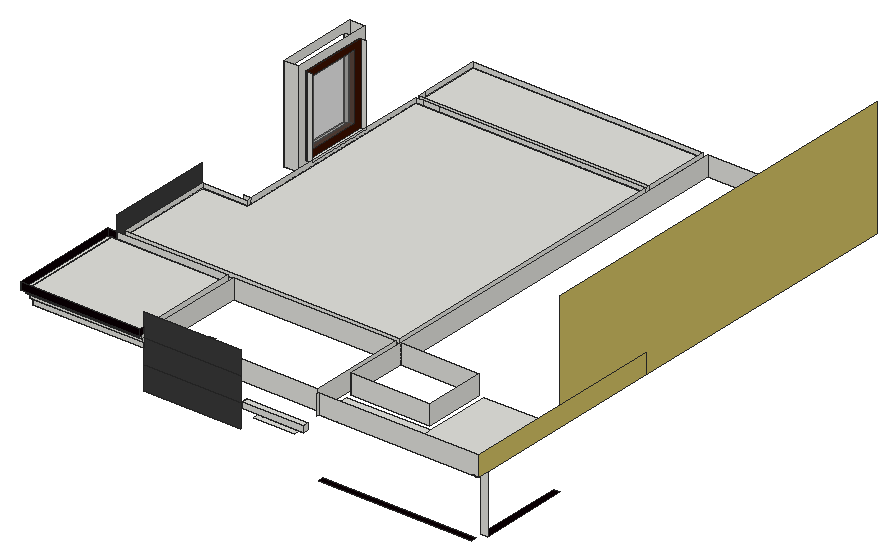
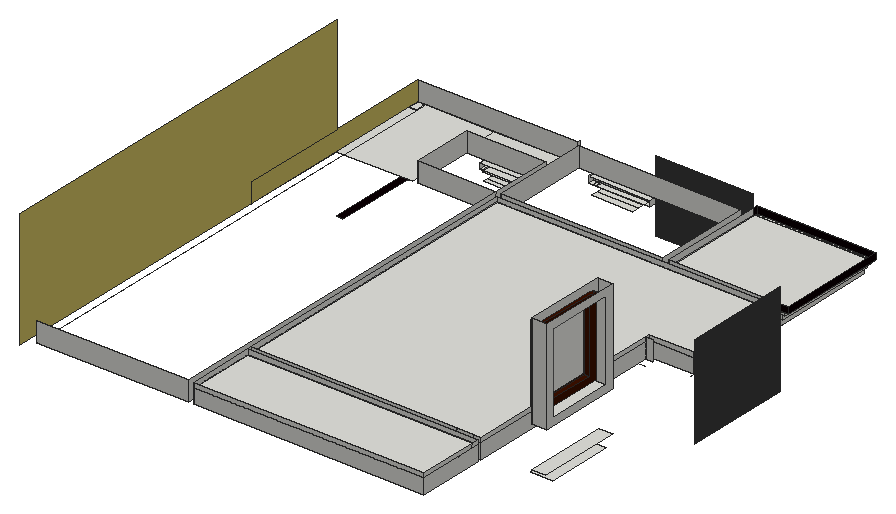
# SketchUp Ruby script. Lengths in inches.
U = 1.inch
M = Sketchup.active_model
def pt(a) = Geom::Point3d.new(a.map { |v| v * U })
def face(e, loops, mat)
  f = e.add_face(loops[0].map { |a| pt(a) })
  loops[1..].each { |l| e.add_face(l.map { |a| pt(a) }).erase! }
  f.material = f.back_material = mat if mat
  f
end
# faces: each face lists its corners as indices into pts; further lists are holes
def faces(e, pts, list, mat = nil) = list.each { |f| face(e, (f[0].is_a?(Array) ? f : [f]).map { |l| l.map { |i| pts[i] } }, mat) }
# xy, xz, yz: faces in a plane at the given z, y or x. An outline is a flat list of corners, or four numbers for a rectangle; further outlines are holes
def ring(l) = l.size == 4 ? [[l[0], l[1]], [l[2], l[1]], [l[2], l[3]], [l[0], l[3]]] : l.each_slice(2).to_a
def flat(e, list, mat, &to3) = list.each { |f| face(e, (f[0].is_a?(Array) ? f : [f]).map { |l| ring(l).map { |u, v| to3.(u, v) } }, mat) }
def xy(e, z, list, mat = nil) = flat(e, list, mat) { |x, y| [x, y, z] }
def xz(e, y, list, mat = nil) = flat(e, list, mat) { |x, z| [x, y, z] }
def yz(e, x, list, mat = nil) = flat(e, list, mat) { |y, z| [x, y, z] }
def lines(e, pts, list) = list.each { |a, b| e.add_line(pt(pts[a]), pt(pts[b])) }
# prism: a flat outline (further loops are holes) pulled along v
def prism(e, loops, v, mat = nil)
  f = face(e, loops, mat); d = Geom::Vector3d.new(v.map { |x| x * U })
  f.pushpull(f.normal.samedirection?(d) ? d.length : -d.length)
end
def box(e, o, s, mat = nil) = prism(e, [[o, [o[0] + s[0], o[1], o[2]], [o[0] + s[0], o[1] + s[1], o[2]], [o[0], o[1] + s[1], o[2]]]], [0, 0, s[2]], mat)
def at(x, y, z, deg = 0) = Geom::Transformation.translation(pt([x, y, z])) * Geom::Transformation.rotation(ORIGIN, Z_AXIS, deg.degrees)
def axes(o, x, y, z) = Geom::Transformation.new([*x, 0, *y, 0, *z, 0, *pt(o).to_a, 1])
def part(name) = M.definitions.add(name)
# library, detail: a bought-in or finely detailed component or shape, given as its bounding box
def library(name, o, s) = part(name).tap { |d| box(d.entities, o, s) }
def detail(e, o, s) = box(e.add_group.entities, o, s)
def put(e, d, t, mat = nil) = e.add_instance(d, t).tap { |i| i.material = mat if mat }
def group(e, t, mat = nil) = e.add_group.tap { |g| g.transformation = t; g.material = mat if mat }.entities
root = M.entities
M.materials.add("[Color C08]").color = [60, 17, 0]
M.materials.add("[Color D05]").color = [208, 191, 99]
M.materials.add("[Color M07]").color = [58, 58, 58]
M.materials.add("[Metal Seamed]").color = [11, 0, 4]
M.materials.add("[Translucent Glass Gray]").color = [128, 128, 128]
M.materials["[Translucent Glass Gray]"].alpha = 0.5
c1 = part("Group\#2")
xy(c1.entities,0,[[0,0,43.625,4]],"[Color C08]")
xy(c1.entities,4.9,[[4.9,0,38.73,4]],"[Color C08]")
xy(c1.entities,53.48,[[4.9,0,38.73,4]],"[Color C08]")
xy(c1.entities,58.375,[[0,0,43.625,4]],"[Color C08]")
xz(c1.entities,0,[[[0,0,43.625,58.375],[4.9,4.9,38.73,53.48]]],"[Color C08]")
xz(c1.entities,0,[[4.9,4.9,38.73,53.48]],"[Translucent Glass Gray]")
xz(c1.entities,4,[[[0,0,43.625,58.375],[4.9,4.9,38.73,53.48]]],"[Color C08]")
yz(c1.entities,0,[[0,0,4,58.375]],"[Color C08]")
yz(c1.entities,4.9,[[0,4.9,4,53.48]],"[Color C08]")
yz(c1.entities,38.73,[[0,4.9,4,53.48]],"[Color C08]")
yz(c1.entities,43.625,[[0,0,4,58.375]],"[Color C08]")
xy(root,191.0625,[[559.49,92.73,560.01,92.74,560.51,92.9,560.95,93.18,561.31,93.56,561.55,94.02,561.67,94.53,561.65,95.05,561.49,95.55,561.22,95.99,560.83,96.35,560.37,96.59,559.86,96.71,559.34,96.6875,558.84,96.53,558.4,96.26,558.04,95.875,557.8,95.41,557.68,94.9,557.7,94.38,557.86,93.88,558.14,93.44,558.52,93.09,558.98,92.84]])
xy(root,192,[[369.3125,70.41,556.3125,77.3]],"[Metal Seamed]")
xy(root,192.96,[[556.24,84.63,564.3125,195.41]],"[Metal Seamed]")
xy(root,216.84,[[55.1875,419.61,72.6875,501.8],[72.6875,419.61,81.6875,501.8]])
xy(root,227.14,[[55.1875,409.31,72.6875,512.1]])
xy(root,232.4375,[[158,120.11,165.5625,168.11]])
xy(root,239.79,[[297.45,60.85,347.52,67.28],[297.45,67.28,347.52,76.28]])
xy(root,239.92,[[395.02,106.41,445.08,113.66],[395.02,113.66,445.08,119.66]])
xy(root,245.34,[[291.9,60.85,349.28,67.28],[349.28,60.85,353.07,67.28]])
xy(root,245.63,[[283.19,59.85,289.58,67.28],[289.58,59.85,349.28,67.28],[349.28,59.85,359.01,60.85],[353.07,60.85,359.01,67.28]])
xy(root,245.96,[[388.97,106.41,451.12,113.66]])
xy(root,246.98,[[385.19,101.28,391.58,113.66],[451.27,101.28,455.06,113.66]])
xy(root,247.26,[[391.58,101.28,451.27,113.66]])
xy(root,252.66,[[283.19,59.85,359.01,67.28]])
xy(root,254.29,[[385.19,101.28,455.06,113.66]])
xy(root,263.5625,[[24.07,73.08,41.19,92.83]])
xy(root,264,[[21.625,67.66,158,195.41],[556.3,70.41,556.3,70.97,555.3125,70.97,555.3125,195.41,564.5,195.41,564.5,84.63,564.3125,84.63,564.3125,70.41],[369.3125,70.97,471.3125,113.66],[471.3125,70.97,555.3125,195.41],[564.3125,195.41,564.5,326.53]])
xy(root,264.0625,[[556.3,70.41,564.3125,70.97],[556.3,70.97,564.3125,70.97,564.3125,84.63,556.24,84.63,556.3,77.3],[564.3125,70.97,564.5,84.63]])
xy(root,271.375,[[19,65.66,19,195.41,21.625,195.41,21.625,67.66,21.75,67.66,21.75,65.66],[21.75,65.66,158,67.66],[21.625,67.66,158,195.41]])
xy(root,276.0625,[[15.8125,63.72,15.8125,195.41,19,195.41,19,65.66,21.75,65.66,21.75,63.72],[21.75,63.72,158,65.66]])
xy(root,276.58,[[55.1875,410.35,72.6875,511.06]])
xy(root,279.875,[[11.6875,61.03,11.6875,67.28,15.8125,67.28,15.8125,63.72,158,63.72,158,61.03],[15.8125,63.72,158,195.41],[11.6875,67.28,15.8125,195.41]])
xy(root,282,[[26.75,201.41,26.75,320.85,81.6875,320.85,81.6875,578.04,363.3125,578.04,363.3125,201.41],[81.6875,582.91,363.3125,665.75]])
xy(root,285.84,[[55.1875,419.61,72.6875,501.8],[72.6875,419.61,81.6875,501.8]])
xz(root,59.85,[[283.19,245.63,359.01,252.66]])
xz(root,60.85,[[349.28,245.34,353.07,245.63]])
xz(root,61.03,[[11.6875,279.875,158,288]],"[Metal Seamed]")
xz(root,63.72,[[15.8125,276.0625,158,279.875]])
xz(root,65.66,[[19,271.375,158,276.0625]])
xz(root,67.28,[[158,217.0625,275.92,246.125],[158,246.125,275.92,275.1875],[158,275.1875,275.92,304.25]],"[Color M07]")
xz(root,67.66,[[21.625,264,158,271.375]])
xz(root,70.41,[[556.3,264,564.3125,264.0625]])
xz(root,70.97,[[369.3125,264,556.3,264,556.3,264.0625,564.5,264.0625,564.5,288,369.3125,288]])
xz(root,76.28,[[165.5625,264,363.3125,288]])
xz(root,84.63,[[556.24,192.96,564.3125,264.0625],[564.3125,264,564.5,264.0625]])
xz(root,101.28,[[385.19,246.98,391.58,246.98,391.58,247.26,451.27,247.26,451.27,246.98,455.06,246.98,455.06,254.29,385.19,254.29]])
xz(root,119.66,[[369.3125,264,465.3125,288]])
xz(root,195.41,[[21.625,264,21.75,271.375],[165.5625,264,363.3125,288],[369.3125,264,465.3125,288],[19,271.375,21.75,276.0625],[21.75,271.375,158,276.0625],
  [15.8125,276.0625,21.75,279.875],[21.75,276.0625,158,279.875],[21.75,279.875,158,288]])
xz(root,195.41,[[11.6875,279.875,21.75,288]],"[Metal Seamed]")
xz(root,201.41,[[26.75,264,363.3125,282],[26.75,282,363.3125,288]])
xz(root,320.85,[[26.75,264,81.6875,282],[26.75,282,81.6875,288]])
xz(root,326.53,[[72.6875,264,81.6875,288],[564.3125,264,564.5,288]])
xz(root,410.35,[[55.1875,276.58,72.6875,392.6]])
xz(root,419.61,[[55.1875,285.84,72.6875,383.34],[72.6875,285.84,81.6875,383.34]])
xz(root,501.8,[[55.1875,285.84,72.6875,383.34],[72.6875,285.84,81.6875,383.34]])
xz(root,511.06,[[55.1875,276.58,72.6875,392.6]])
xz(root,578.04,[[81.6875,264,363.3125,282],[81.6875,282,90.52,288],[90.52,282,111.08,288],[111.08,282,363.3125,288]])
xz(root,582.91,[[81.6875,264,363.3125,282],[81.6875,282,363.3125,288]])
xz(root,664.97,[[369.3125,264,555.3125,288]])
xz(root,665.75,[[81.6875,264,363.3125,282],[81.6875,282,363.3125,288]])
yz(root,11.6875,[[61.03,279.875,195.41,288]],"[Metal Seamed]")
yz(root,15.8125,[[63.72,276.0625,195.41,279.875]])
yz(root,19,[[65.66,271.375,195.41,276.0625]])
yz(root,21.625,[[67.66,264,195.41,271.375]])
yz(root,21.75,[[195.41,191.53,326.53,220.09],[195.41,220.09,326.53,248.65],[195.41,248.65,326.53,277.22],[195.41,277.22,326.53,305.78]],"[Color M07]")
yz(root,26.75,[[201.41,264,320.85,282],[201.41,282,320.85,288]])
yz(root,55.1875,[[[410.35,276.58,511.06,392.6],[419.61,285.84,501.8,383.34]]])
yz(root,72.6875,[[[410.35,276.58,511.06,392.6],[419.61,285.84,501.8,383.34]]])
yz(root,81.6875,[[320.85,264,326.53,282],[326.53,264,578.04,282],[582.91,264,665.75,282],[320.85,282,326.53,288],[326.53,282,578.04,282,578.04,288,501.8,288,501.8,285.84,419.61,285.84,419.61,288,326.53,288],
  [582.91,282,592.78,288],[592.78,282,665.75,288],[419.61,285.84,501.8,288]])
yz(root,158,[[67.28,264,67.66,271.375],[65.66,271.375,67.28,276.0625],[67.28,271.375,195.41,276.0625],[63.72,276.0625,67.28,279.875],[67.28,276.0625,195.41,279.875],
  [67.28,279.875,195.41,288]])
yz(root,158,[[61.03,279.875,67.28,288]],"[Metal Seamed]")
yz(root,165.5625,[[76.28,264,195.41,288]])
yz(root,283.19,[[59.85,245.63,67.28,252.66]])
yz(root,349.28,[[60.85,245.34,67.28,245.63]])
yz(root,353.07,[[60.85,245.34,67.28,245.63]])
yz(root,359.01,[[59.85,245.63,67.28,252.66]])
yz(root,363.3125,[[76.28,264,195.41,288],[201.41,264,578.04,282],[578.04,264,582.91,288],[582.91,264,665.75,282],[201.41,282,578.04,288],
  [582.91,282,665.75,288]])
yz(root,369.3125,[[67.28,264,70.97,288],[119.66,264,195.41,288],[195.41,264,664.97,288]])
yz(root,385.19,[[101.28,246.98,113.66,254.29]])
yz(root,391.58,[[101.28,246.98,113.66,247.26]])
yz(root,451.27,[[101.28,246.98,113.66,247.26]])
yz(root,455.06,[[101.28,246.98,113.66,254.29]])
yz(root,465.3125,[[119.66,264,195.41,288]])
yz(root,556.3,[[70.41,264,70.97,264.0625]])
yz(root,564.3125,[[70.41,264,84.63,264.0625]])
yz(root,564.3125,[[326.53,264,679.25,264,679.25,408,195.41,408,195.41,288,326.53,288]],"[Color D05]")
yz(root,564.5,[[84.63,264,326.53,264,326.53,288,70.97,288,70.97,264.0625,84.63,264.0625]],"[Color D05]")
p = [[555.3125,195.41,264],[555.3125,664.97,264],[81.6875,338.22,264],[72.6875,338.22,264],[26.75,320.85,264],[26.75,326.53,264]]
lines(root,p,[[0,1],[2,3],[4,5]])
put(root,c1,axes([75.57,501.8,285.84],[0,-1.88395,0],[-1.8,0,0],[0,0,1.67024]))
